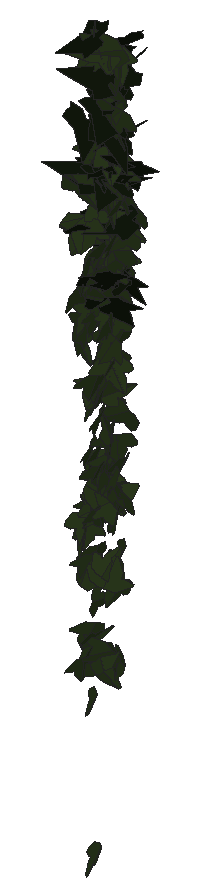
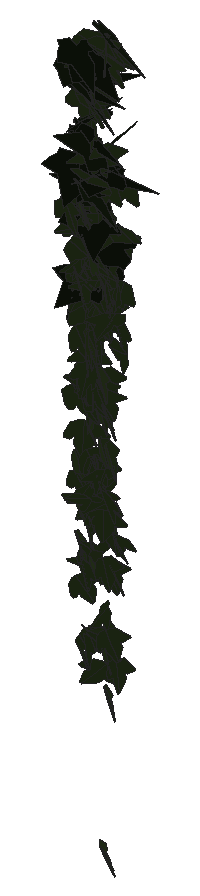
# SketchUp Ruby script. Lengths in inches.
U = 1.inch
M = Sketchup.active_model
def pt(a) = Geom::Point3d.new(a.map { |v| v * U })
def face(e, loops, mat)
  f = e.add_face(loops[0].map { |a| pt(a) })
  loops[1..].each { |l| e.add_face(l.map { |a| pt(a) }).erase! }
  f.material = f.back_material = mat if mat
  f
end
# faces: each face lists its corners as indices into pts; further lists are holes
def faces(e, pts, list, mat = nil) = list.each { |f| face(e, (f[0].is_a?(Array) ? f : [f]).map { |l| l.map { |i| pts[i] } }, mat) }
# xy, xz, yz: faces in a plane at the given z, y or x. An outline is a flat list of corners, or four numbers for a rectangle; further outlines are holes
def ring(l) = l.size == 4 ? [[l[0], l[1]], [l[2], l[1]], [l[2], l[3]], [l[0], l[3]]] : l.each_slice(2).to_a
def flat(e, list, mat, &to3) = list.each { |f| face(e, (f[0].is_a?(Array) ? f : [f]).map { |l| ring(l).map { |u, v| to3.(u, v) } }, mat) }
def xy(e, z, list, mat = nil) = flat(e, list, mat) { |x, y| [x, y, z] }
def xz(e, y, list, mat = nil) = flat(e, list, mat) { |x, z| [x, y, z] }
def yz(e, x, list, mat = nil) = flat(e, list, mat) { |y, z| [x, y, z] }
def lines(e, pts, list) = list.each { |a, b| e.add_line(pt(pts[a]), pt(pts[b])) }
# prism: a flat outline (further loops are holes) pulled along v
def prism(e, loops, v, mat = nil)
  f = face(e, loops, mat); d = Geom::Vector3d.new(v.map { |x| x * U })
  f.pushpull(f.normal.samedirection?(d) ? d.length : -d.length)
end
def box(e, o, s, mat = nil) = prism(e, [[o, [o[0] + s[0], o[1], o[2]], [o[0] + s[0], o[1] + s[1], o[2]], [o[0], o[1] + s[1], o[2]]]], [0, 0, s[2]], mat)
def at(x, y, z, deg = 0) = Geom::Transformation.translation(pt([x, y, z])) * Geom::Transformation.rotation(ORIGIN, Z_AXIS, deg.degrees)
def axes(o, x, y, z) = Geom::Transformation.new([*x, 0, *y, 0, *z, 0, *pt(o).to_a, 1])
def part(name) = M.definitions.add(name)
# library, detail: a bought-in or finely detailed component or shape, given as its bounding box
def library(name, o, s) = part(name).tap { |d| box(d.entities, o, s) }
def detail(e, o, s) = box(e.add_group.entities, o, s)
def put(e, d, t, mat = nil) = e.add_instance(d, t).tap { |i| i.material = mat if mat }
def group(e, t, mat = nil) = e.add_group.tap { |g| g.transformation = t; g.material = mat if mat }.entities
root = M.entities
M.materials.add("1026 AP 7946 SUNNY SIDE UP").color = [254, 231, 186]
M.materials.add("efeu1").color = [18, 25, 13]
M.materials.add("efeu2").color = [43, 57, 29]
c1 = part("ivyleaf_10")
p = [[0,0.5,-0.03],[-0.0625,2.02,-0.43],[-0.19,2.01,-0.46],[-0.54,1.05,-0.29],[-0.52,0.625,-0.18],[-0.83,0.76,-0.28],
  [-1.16,0.64,-0.33],[-1.15,0.33,-0.24],[-0.77,-0.39,0.02],[-0.3,-0.51,0.16],[0.04,-0.48,0.23],[-0.02,2.01,-0.4375],
  [-0.06,2.01,-0.43],[0.04,-0.49,0.23],[0.67,-0.49,0.14],[1.38,0.36,-0.2],[1.375,0.51,-0.24],[0.81,0.65,-0.19],
  [0.62,0.59,-0.15],[0.6,1.09,-0.28],[0.5,1.23,-0.31]]
faces(c1.entities,p,[[0,1,2,3,4,5,6,7,8,9,10],[11,12,0,13,14,15,16,17,18,19,20]],"efeu2")
c2 = part("ivyleaf_9")
p = [[1.54,2.16,1.25],[1.36,2.04,1.19],[-0.21,0.99,0.68],[-0.71,1.11,0.82],[-0.85,0.86,0.67],[-0.8,0.17,0.21],
  [-0.9,-0.01,0.1],[-0.67,-0.16,-0.02],[-0.08,-0.08,-0.05],[-0.03,-0.6,-0.4],[0.65,-0.88,-0.66],[0.83,-0.6,-0.49],
  [1.29,-0.42,-0.43],[1.8125,-0.07,-0.26],[1.21,0.44,0.15]]
faces(c2.entities,p,[[0,1,2,3,4,5,6,7,8,9,10,11,12,13,14]],"efeu1")
put(root,c1,axes([98.29,212.76,264.19],[-0.22971,-0.152,0.11857],[-0.04918,-0.12497,-0.21008],[0.29657,-0.13846,0.057]),"1026 AP 7946 SUNNY SIDE UP")
put(root,c1,axes([98.25,213.08,261.87],[0.0644,-0.18084,-0.07279],[-0.03638,0.06251,-0.19678],[0.32455,0.04289,-0.00761]),"1026 AP 7946 SUNNY SIDE UP")
put(root,c1,axes([98.24,212.66,256.42],[-0.06854,-0.19891,-0.02661],[0.0175,0.02284,-0.20955],[0.31468,-0.04459,0.00586]),"1026 AP 7946 SUNNY SIDE UP")
put(root,c1,axes([98.11,212.79,258.72],[0.18384,-0.12088,0.13408],[0.13954,-0.09617,-0.17379],[0.24285,0.14677,-0.00164]),"1026 AP 7946 SUNNY SIDE UP")
put(root,c1,axes([98.26,212.58,262.52],[0.22707,-0.1538,-0.09871],[-0.05451,0.0957,-0.21347],[0.27893,0.14391,0.03864]),"1026 AP 7946 SUNNY SIDE UP")
put(root,c1,axes([98.16,212.81,258.85],[0.32191,-0.01328,0.03541],[0.0514,-0.02499,-0.21022],[0.02698,0.20609,-0.02198]),"1026 AP 7946 SUNNY SIDE UP")
put(root,c2,axes([98.14,212.84,266.04],[-0.01817,-0.22293,0.11408],[-0.01715,-0.11156,-0.23057],[0.39191,-0.01522,-0.0048]),"1026 AP 7946 SUNNY SIDE UP")
put(root,c2,axes([98.54,212.66,265.22],[-0.21843,0.05872,0.17567],[-0.27405,0.03415,-0.14884],[-0.10817,-0.2051,0.02234]),"1026 AP 7946 SUNNY SIDE UP")
put(root,c1,axes([98.09,212.75,262.18],[-0.13955,0.04564,-0.21141],[0.16862,-0.18208,-0.09045],[-0.28479,-0.13017,0.05004]),"1026 AP 7946 SUNNY SIDE UP")
put(root,c1,axes([98.29,212.8,258.22],[-0.09401,-0.19406,0.04191],[-0.00495,-0.0427,-0.20922],[0.3121,-0.05913,0.0093]),"1026 AP 7946 SUNNY SIDE UP")
put(root,c1,axes([98.3,212.81,256.99],[-0.12749,-0.17983,0.05348],[-0.01708,-0.05307,-0.20319],[0.29427,-0.08099,0.01138]),"1026 AP 7946 SUNNY SIDE UP")
put(root,c1,axes([98.24,212.52,263.16],[-0.01748,-0.19451,-0.168],[0.06344,0.15869,-0.19825],[0.39292,-0.03427,0.02454]),"1026 AP 7946 SUNNY SIDE UP")
put(root,c1,axes([98.29,212.92,258.35],[-0.0743,-0.19922,0.00153],[0.00432,-0.00334,-0.21091],[0.31325,-0.0472,0.00327]),"1026 AP 7946 SUNNY SIDE UP")
put(root,c1,axes([98.15,212.93,262.87],[0.15264,0.20177,0.06018],[0.05518,0.04659,-0.23011],[-0.32514,0.10263,-0.0108]),"1026 AP 7946 SUNNY SIDE UP")
put(root,c1,axes([98.27,212.92,259.6],[0.24617,-0.13627,-0.02644],[-0.02313,0.021,-0.2136],[0.21659,0.15712,0.00724]),"1026 AP 7946 SUNNY SIDE UP")
put(root,c1,axes([98.27,212.91,263.41],[0.16233,-0.20482,-0.05122],[0.00816,0.05655,-0.23401],[0.33088,0.09909,0.0309]),"1026 AP 7946 SUNNY SIDE UP")
put(root,c1,axes([98.29,212.88,261.1],[0.17184,-0.19541,-0.00772],[-0.00907,0.00409,-0.23061],[0.30729,0.1094,-0.00249]),"1026 AP 7946 SUNNY SIDE UP")
put(root,c1,axes([98.26,212.67,257.9],[0.28096,-0.11428,0.0199],[-0.00721,0.02968,0.21746],[-0.18228,-0.17733,0.02207]),"1026 AP 7946 SUNNY SIDE UP")
put(root,c1,axes([98.34,212.9,259.1875],[-0.23044,-0.1348,-0.00393],[0.02391,-0.01147,-0.20406],[0.2276,-0.13528,0.01745]),"1026 AP 7946 SUNNY SIDE UP")
put(root,c1,axes([98.21,212.58,265.1],[-0.30673,-0.00524,-0.11432],[0.17984,-0.03596,-0.19065],[-0.0235,-0.20674,0.03309]),"1026 AP 7946 SUNNY SIDE UP")
put(root,c1,axes([98.34,212.74,260.3],[0.08197,-0.21019,-0.01942],[-0.00422,0.01752,-0.22299],[0.33164,0.05218,0.00196]),"1026 AP 7946 SUNNY SIDE UP")
put(root,c1,axes([98.32,212.76,263.54],[-0.00491,0.19552,-0.13215],[-0.06305,-0.12793,-0.19892],[-0.36322,0.01956,0.03632]),"1026 AP 7946 SUNNY SIDE UP")
put(root,c1,axes([98.41,212.92,261.34],[-0.23131,-0.1322,0.10215],[-0.04616,-0.11069,-0.19607],[0.25644,-0.13918,0.05685]),"1026 AP 7946 SUNNY SIDE UP")
put(root,c1,axes([98.26,212.66,264.32],[0.37558,0.0164,0.01636],[0.02822,-0.0215,-0.23658],[-0.02517,0.22072,-0.02113]),"1026 AP 7946 SUNNY SIDE UP")
put(root,c1,axes([98.46,212.72,267.62],[-0.15758,0.12687,0.17889],[-0.19353,0.12074,-0.16592],[-0.29632,-0.14632,0.01323]),"1026 AP 7946 SUNNY SIDE UP")
put(root,c1,axes([98.32,212.85,257.47],[0.00636,-0.06188,-0.20073],[0.06148,0.19116,-0.0607],[0.31498,-0.03607,0.0159]),"1026 AP 7946 SUNNY SIDE UP")
put(root,c2,axes([98.57,212.6,267.8],[-0.29349,0.1754,-0.0108],[-0.00675,-0.02125,-0.26328],[-0.29842,-0.17203,0.01658]),"1026 AP 7946 SUNNY SIDE UP")
put(root,c1,axes([98.4,212.84,265.7],[-0.1176,-0.21924,0.09],[0.01541,-0.09572,-0.23605],[0.37151,-0.06543,0.03828]),"1026 AP 7946 SUNNY SIDE UP")
put(root,c1,axes([98.44,212.81,267.4],[0.32445,-0.06472,-0.08538],[-0.13908,0.00256,-0.21468],[0.10328,0.20676,-0.02089]),"1026 AP 7946 SUNNY SIDE UP")
put(root,c1,axes([98.32,212.92,260],[0.10546,0.20612,0.01823],[0.00051,0.01727,-0.22314],[-0.32515,0.06688,0.00557]),"1026 AP 7946 SUNNY SIDE UP")
put(root,c1,axes([98.4,212.76,256.75],[0.06758,-0.19814,-0.01738],[-0.00061,0.01602,-0.20875],[0.31254,0.04287,0.00335]),"1026 AP 7946 SUNNY SIDE UP")
put(root,c2,axes([98.12,212.7,264.03],[0.2292,0.15255,-0.11025],[0.09916,0.08819,0.21888],[0.2983,-0.14653,0.01196]),"1026 AP 7946 SUNNY SIDE UP")
put(root,c1,axes([98.42,212.92,261.49],[-0.0993,-0.20231,0.06325],[0.01792,-0.06842,-0.21653],[0.33248,-0.05673,0.03056]),"1026 AP 7946 SUNNY SIDE UP")
put(root,c1,axes([98.48,212.74,262.78],[-0.16529,-0.15216,0.13866],[-0.05787,-0.13573,-0.18729],[0.31505,-0.10476,0.03834]),"1026 AP 7946 SUNNY SIDE UP")
put(root,c1,axes([98.62,212.72,267.54],[0.20334,-0.01781,-0.20681],[-0.32888,-0.01482,-0.12751],[-0.00553,0.22662,-0.0214]),"1026 AP 7946 SUNNY SIDE UP")
put(root,c1,axes([98.45,212.84,259.18],[0.02115,0.12114,-0.15666],[-0.11695,-0.13542,-0.12685],[-0.30275,0.06077,0.03806]),"1026 AP 7946 SUNNY SIDE UP")
put(root,c2,axes([98.55,213.04,267.42],[-0.01764,0.14972,-0.1576],[-0.0575,-0.1486,-0.15923],[-0.35413,0.01667,0.0337]),"1026 AP 7946 SUNNY SIDE UP")
put(root,c1,axes([98.45,212.94,263.88],[0.0211,-0.2373,0.00856],[-0.01113,-0.01007,-0.24479],[0.37327,0.01311,-0.00778]),"1026 AP 7946 SUNNY SIDE UP")
put(root,c1,axes([98.45,212.65,255.84],[0.12871,-0.1796,-0.04971],[-0.03129,0.04283,-0.20308],[0.29033,0.08424,0.00015]),"1026 AP 7946 SUNNY SIDE UP")
put(root,c1,axes([98.47,212.68,261.59],[-0.08202,-0.216,0.00735],[-0.00232,-0.00825,-0.22897],[0.33989,-0.05218,0.00021]),"1026 AP 7946 SUNNY SIDE UP")
put(root,c1,axes([98.43,212.75,253.03],[0.18468,-0.17561,0.0376],[0.01679,-0.03789,-0.21751],[0.28185,0.11732,-0.01168]),"1026 AP 7946 SUNNY SIDE UP")
put(root,c1,axes([98.48,212.95,263.35],[-0.11362,-0.21292,0.0654],[0.00117,-0.06825,-0.23095],[0.34991,-0.06891,0.02201]),"1026 AP 7946 SUNNY SIDE UP")
put(root,c2,axes([98.67,212.83,266.93],[-0.13402,-0.01059,0.22062],[-0.3224,-0.08292,-0.08356],[0.13757,-0.20465,0.01911]),"1026 AP 7946 SUNNY SIDE UP")
put(root,c1,axes([98.49,212.76,262.75],[-0.00318,-0.22617,0.04436],[0.0058,-0.04437,-0.23323],[0.36235,-0.00127,0.00412]),"1026 AP 7946 SUNNY SIDE UP")
put(root,c1,axes([98.39,212.63,256.82],[0.03832,-0.12765,0.1596],[0.03869,0.1575,0.13002],[-0.31415,0.00383,0.03548]),"1026 AP 7946 SUNNY SIDE UP")
put(root,c1,axes([98.5,212.7,260.34],[0.06741,-0.21819,-0.02668],[-0.00984,0.0239,-0.22893],[0.34512,0.0433,-0.00131]),"1026 AP 7946 SUNNY SIDE UP")
put(root,c1,axes([98.5,212.8,259.97],[-0.2697,0.13388,-0.00878],[-0.00333,-0.01777,-0.2237],[-0.21099,-0.17085,0.01476]),"1026 AP 7946 SUNNY SIDE UP")
put(root,c2,axes([98.41,212.76,265.45],[0.31349,0.13977,0.00154],[0.02054,-0.01661,-0.2472],[-0.23637,0.18392,-0.01943]),"1026 AP 7946 SUNNY SIDE UP")
put(root,c2,axes([98.68,212.85,265.05],[-0.1762,0.19802,-0.02045],[-0.00038,-0.02457,-0.23938],[-0.33816,-0.10315,0.01093]),"1026 AP 7946 SUNNY SIDE UP")
put(root,c1,axes([98.46,212.87,264.55],[0.20199,0.18711,-0.02128],[-0.01911,-0.01929,-0.23766],[-0.31931,0.11952,0.00076]),"1026 AP 7946 SUNNY SIDE UP")
put(root,c1,axes([98.43,212.98,263.4],[0.20222,0.17425,0.02367],[0.03433,0.01017,-0.22553],[-0.29572,0.12034,-0.01]),"1026 AP 7946 SUNNY SIDE UP")
put(root,c1,axes([98.46,212.63,259.61],[0.00453,0.1569,0.18599],[0.00817,0.17957,-0.16061],[-0.37495,0.00581,-0.00125]),"1026 AP 7946 SUNNY SIDE UP")
put(root,c1,axes([98.53,212.88,258.31],[0.09902,-0.18601,0.06887],[0.01632,-0.06806,-0.20237],[0.31094,0.06281,-0.01131]),"1026 AP 7946 SUNNY SIDE UP")
put(root,c1,axes([98.31,212.69,263.01],[-0.16068,0.05872,0.20743],[0.31684,-0.05539,0.11527],[0.12993,0.20769,-0.02457]),"1026 AP 7946 SUNNY SIDE UP")
put(root,c1,axes([98.35,212.85,259.41],[0.16698,0.11056,0.17086],[0.15036,0.13582,-0.15615],[-0.27406,0.14188,0.01843]),"1026 AP 7946 SUNNY SIDE UP")
put(root,c1,axes([98.54,212.77,260.05],[0.07045,-0.20519,-0.05876],[0.00231,0.05739,-0.2156],[0.33437,0.04283,0.01387]),"1026 AP 7946 SUNNY SIDE UP")
put(root,c2,axes([98.74,212.79,266.62],[-0.13603,0.17689,0.13039],[-0.09173,0.10667,-0.20636],[-0.35056,-0.09655,0.0034]),"1026 AP 7946 SUNNY SIDE UP")
put(root,c1,axes([98.79,212.75,267.59],[-0.18146,-0.02474,0.21694],[-0.30435,-0.09875,-0.11536],[0.16684,-0.20704,0.02552]),"1026 AP 7946 SUNNY SIDE UP")
put(root,c1,axes([98.49,212.72,265.05],[-0.34821,0.02393,-0.05338],[0.08016,-0.02618,-0.22042],[-0.04978,-0.20954,0.01843]),"1026 AP 7946 SUNNY SIDE UP")
put(root,c1,axes([98.54,212.69,259.25],[-0.0547,-0.1988,-0.06869],[0.03334,0.06276,-0.20732],[0.32746,-0.0396,0.00963]),"1026 AP 7946 SUNNY SIDE UP")
put(root,c1,axes([98.55,213,262.38],[0.13716,-0.20864,-0.00904],[-0.00331,0.00734,-0.23292],[0.32826,0.08725,0.00143]),"1026 AP 7946 SUNNY SIDE UP")
put(root,c2,axes([98.56,212.88,264.54],[0.22407,0.15525,-0.0973],[-0.08442,-0.07945,-0.21887],[-0.29531,0.14051,-0.01126]),"1026 AP 7946 SUNNY SIDE UP")
put(root,c1,axes([98.8,212.78,266.64],[-0.14241,0.01609,-0.22262],[-0.31485,0.09723,0.08943],[0.16268,0.20226,-0.02179]),"1026 AP 7946 SUNNY SIDE UP")
put(root,c1,axes([98.75,212.6,256.8],[-0.21755,-0.02541,0.16831],[-0.24391,-0.05432,-0.14423],[0.09063,-0.2072,0.01586]),"1026 AP 7946 SUNNY SIDE UP")
put(root,c1,axes([98.54,212.91,263.25],[-0.05203,-0.19356,0.12847],[0.05525,-0.12983,-0.19703],[0.35877,-0.00808,0.04898]),"1026 AP 7946 SUNNY SIDE UP")
put(root,c1,axes([98.29,212.87,263.54],[-0.01317,-0.03736,-0.21087],[0.30872,-0.08315,0.00808],[-0.1413,-0.17819,0.03731]),"1026 AP 7946 SUNNY SIDE UP")
put(root,c1,axes([98.66,212.63,259.4],[0.25898,-0.03648,-0.11675],[-0.18808,-0.0011,-0.16628],[0.04935,0.18726,-0.02101]),"1026 AP 7946 SUNNY SIDE UP")
put(root,c1,axes([98.62,212.76,262.41],[0.19891,-0.13599,-0.13967],[-0.0746,0.13427,-0.18462],[0.2917,0.12707,0.04802]),"1026 AP 7946 SUNNY SIDE UP")
put(root,c2,axes([98.83,212.875,266.02],[-0.07929,-0.01751,-0.23],[-0.35915,-0.03705,0.05202],[-0.06788,0.21648,-0.00657]),"1026 AP 7946 SUNNY SIDE UP")
put(root,c1,axes([98.56,213,261.82],[-0.16417,-0.18385,-0.07249],[0.06126,0.05757,-0.21741],[0.30281,-0.11132,0.00469]),"1026 AP 7946 SUNNY SIDE UP")
put(root,c1,axes([98.57,212.93,262.33],[0.0441,-0.22086,-0.0545],[0.0189,0.05341,-0.22828],[0.35615,0.02451,0.01886]),"1026 AP 7946 SUNNY SIDE UP")
put(root,c1,axes([98.56,212.96,263.54],[0.34388,-0.06462,-0.01762],[-0.03387,-0.01132,-0.22709],[0.10764,0.20286,-0.01515]),"1026 AP 7946 SUNNY SIDE UP")
put(root,c1,axes([98.59,212.65,261],[0.07606,-0.21281,-0.02731],[-0.00535,0.02518,-0.22466],[0.33693,0.04844,0.0026]),"1026 AP 7946 SUNNY SIDE UP")
put(root,c1,axes([98.625,212.93,263.56],[-0.29347,-0.13998,0.02087],[-0.00932,-0.02708,-0.23978],[0.22238,-0.18586,0.01749]),"1026 AP 7946 SUNNY SIDE UP")
put(root,c1,axes([98.59,212.69,259.99],[-0.14589,-0.19351,-0.03192],[0.02549,0.02536,-0.2209],[0.30683,-0.09412,0.00318]),"1026 AP 7946 SUNNY SIDE UP")
put(root,c1,axes([98.83,212.95,263.91],[-0.16824,0.02149,0.21702],[-0.33044,-0.03867,-0.10618],[0.03933,-0.23298,0.03623]),"1026 AP 7946 SUNNY SIDE UP")
put(root,c1,axes([98.48,212.77,256.35],[-0.23899,-0.05882,-0.10548],[0.1652,0.01912,-0.16209],[0.10107,-0.17033,0.01554]),"1026 AP 7946 SUNNY SIDE UP")
put(root,c2,axes([98.87,212.97,266.875],[-0.20248,0.08561,0.17261],[-0.24506,0.07146,-0.15504],[-0.18691,-0.18643,0.0163]),"1026 AP 7946 SUNNY SIDE UP")
put(root,c2,axes([98.73,212.68,264.93],[-0.13027,0.21192,-0.06355],[0.02841,-0.06,-0.24209],[-0.37381,-0.07841,0.00375]),"1026 AP 7946 SUNNY SIDE UP")
put(root,c2,axes([98.81,212.92,263.43],[-0.31796,0.10225,-0.00173],[-0.02754,-0.03576,-0.22508],[-0.17146,-0.18388,0.03936]),"1026 AP 7946 SUNNY SIDE UP")
put(root,c1,axes([98.62,212.71,261.46],[0.04827,-0.18386,-0.12807],[0.01233,0.12528,-0.18974],[0.34785,0.02107,0.0245]),"1026 AP 7946 SUNNY SIDE UP")
put(root,c1,axes([98.69,212.82,266.11],[-0.26979,0.14287,0.07169],[-0.10595,0.02751,-0.22737],[-0.24456,-0.16953,0.01941]),"1026 AP 7946 SUNNY SIDE UP")
put(root,c1,axes([98.63,212.94,259.07],[0.17358,-0.16747,-0.06473],[-0.02321,0.06394,-0.20504],[0.27977,0.10921,0.02315]),"1026 AP 7946 SUNNY SIDE UP")
put(root,c1,axes([98.52,212.91,259.47],[-0.0039,-0.03391,0.20392],[0.06767,0.18677,0.03863],[-0.32214,0.03965,0.00565]),"1026 AP 7946 SUNNY SIDE UP")
put(root,c1,axes([98.61,212.79,261.66],[0.18076,-0.18083,0.03539],[0.02664,-0.03186,-0.22509],[0.31166,0.1076,-0.00129]),"1026 AP 7946 SUNNY SIDE UP")
put(root,c2,axes([98.72,213.07,267.63],[-0.00026,0.20628,-0.07428],[0.00297,-0.07207,-0.22184],[-0.37092,-0.00072,-0.00172]),"1026 AP 7946 SUNNY SIDE UP")
put(root,c2,axes([98.53,212.83,265.76],[-0.02895,0.20921,-0.09732],[-0.01141,0.09339,0.22602],[0.38892,0.01831,-0.00062]),"1026 AP 7946 SUNNY SIDE UP")
put(root,c1,axes([98.81,212.96,264.77],[-0.12362,0.08842,0.1741],[-0.25298,0.07363,-0.11409],[-0.18347,-0.1611,0.04002]),"1026 AP 7946 SUNNY SIDE UP")
put(root,c1,axes([98.68,212.79,260.11],[-0.11545,-0.18541,0.08634],[0.00568,-0.09136,-0.20296],[0.32057,-0.06516,0.03469]),"1026 AP 7946 SUNNY SIDE UP")
put(root,c1,axes([98.68,213.04,259.4375],[0.19254,0.14351,0.03527],[-0.0485,-0.01695,0.19519],[0.2445,-0.11638,0.01094]),"1026 AP 7946 SUNNY SIDE UP")
put(root,c1,axes([98.7,212.81,259.66],[0.27995,-0.07665,-0.08339],[-0.0837,0.07467,-0.19407],[0.15345,0.18057,0.04628]),"1026 AP 7946 SUNNY SIDE UP")
put(root,c1,axes([98.78,212.49,256.61],[0.20979,0.01129,0.17228],[-0.22548,0.12189,0.10184],[-0.15497,-0.16207,0.08504]),"1026 AP 7946 SUNNY SIDE UP")
put(root,c1,axes([98.68,212.89,264.12],[0.1125,-0.22648,0.01529],[0.00214,-0.01648,-0.24475],[0.35701,0.07147,-0.00335]),"1026 AP 7946 SUNNY SIDE UP")
put(root,c2,axes([98.63,212.92,265.22],[-0.15691,-0.20919,0.08344],[-0.00227,-0.08932,-0.23655],[0.35339,-0.09345,0.03553]),"1026 AP 7946 SUNNY SIDE UP")
put(root,c1,axes([98.75,212.84,267.19],[0.21967,-0.18607,-0.14023],[-0.08683,0.12626,-0.2373],[0.35095,0.14771,0.02906]),"1026 AP 7946 SUNNY SIDE UP")
put(root,c1,axes([98.71,212.71,260.65],[-0.10821,0.19681,0.01786],[0.01391,-0.01219,0.22126],[0.33466,0.06415,-0.00342]),"1026 AP 7946 SUNNY SIDE UP")
put(root,c2,axes([98.61,212.82,266.36],[-0.11875,-0.19783,0.13988],[0.01707,-0.14615,-0.21225],[0.37791,-0.05556,0.05354]),"1026 AP 7946 SUNNY SIDE UP")
put(root,c1,axes([98.63,212.83,265.61],[0.17086,0.19212,-0.02318],[-0.00369,-0.0261,-0.2323],[-0.32867,0.10016,-0.00944]),"1026 AP 7946 SUNNY SIDE UP")
put(root,c1,axes([98.78,212.79,266.63],[0.23094,-0.15536,-0.1016],[-0.12471,0.05879,-0.21967],[0.28082,0.15387,-0.014]),"1026 AP 7946 SUNNY SIDE UP")
put(root,c1,axes([98.73,212.96,261.65],[0.03055,-0.22032,-0.0356],[-0.0079,0.03299,-0.22765],[0.35027,0.01996,-0.00203]),"1026 AP 7946 SUNNY SIDE UP")
put(root,c2,axes([98.64,212.47,263.5625],[0.22787,0.16303,0.03021],[0.04484,0.01198,-0.22551],[-0.27666,0.13622,-0.01167]),"1026 AP 7946 SUNNY SIDE UP")
put(root,c1,axes([98.56,212.96,265.25],[0.34479,0.06424,0.07957],[0.11629,0.02098,-0.23527],[-0.10626,0.23141,0.00071]),"1026 AP 7946 SUNNY SIDE UP")
put(root,c1,axes([98.67,212.8,264.37],[0.37011,0.06859,-0.0088],[0.00183,0.02775,0.25127],[0.10875,-0.23391,0.02572]),"1026 AP 7946 SUNNY SIDE UP")
put(root,c1,axes([98.75,212.84,262.74],[-0.22899,-0.15956,0.08321],[0.01391,-0.11151,-0.20882],[0.28152,-0.12428,0.07801]),"1026 AP 7946 SUNNY SIDE UP")
put(root,c1,axes([98.75,212.98,262.4],[-0.06608,-0.21769,0.05134],[-0.00053,-0.0519,-0.22851],[0.35159,-0.04099,0.0093]),"1026 AP 7946 SUNNY SIDE UP")
put(root,c1,axes([98.73,212.91,264.71],[0.12622,-0.22115,0.06583],[0.0117,-0.06647,-0.24226],[0.36233,0.07918,-0.01511]),"1026 AP 7946 SUNNY SIDE UP")
put(root,c1,axes([98.7,212.93,258.22],[0.24763,-0.134,-0.01358],[0.01432,0.02969,-0.21082],[0.21112,0.15516,0.03023]),"1026 AP 7946 SUNNY SIDE UP")
put(root,c1,axes([98.68,212.77,264.86],[-0.04794,0.20085,-0.04463],[0.00065,-0.04467,-0.21768],[-0.34914,-0.02766,0.00572]),"1026 AP 7946 SUNNY SIDE UP")
put(root,c1,axes([98.78,212.93,257.88],[-0.10308,-0.16725,0.09671],[-0.01814,-0.09659,-0.18427],[0.30177,-0.06294,0.02196]),"1026 AP 7946 SUNNY SIDE UP")
put(root,c2,axes([98.51,212.73,265.1],[0.12238,0.03821,0.20927],[0.30645,0.07404,-0.08596],[-0.14088,0.19425,-0.00519]),"1026 AP 7946 SUNNY SIDE UP")
put(root,c1,axes([98.72,212.66,263.63],[-0.13153,-0.20394,-0.09686],[0.07172,0.08155,-0.22635],[0.34497,-0.09471,0.01013]),"1026 AP 7946 SUNNY SIDE UP")
put(root,c1,axes([98.77,212.75,262],[0.03354,-0.15201,-0.11535],[-0.02207,0.10496,-0.16265],[0.31359,0.02365,0.00089]),"1026 AP 7946 SUNNY SIDE UP")
put(root,c1,axes([98.7,212.65,259.98],[0.03428,-0.18912,-0.11405],[0.07805,0.11158,-0.18747],[0.33475,-0.00665,0.05539]),"1026 AP 7946 SUNNY SIDE UP")
put(root,c1,axes([98.81,212.71,266.5],[-0.3906,0.04949,0.02491],[-0.05289,-0.03922,-0.24794],[-0.07573,-0.22786,0.04466]),"1026 AP 7946 SUNNY SIDE UP")
put(root,c1,axes([98.69,212.9375,263.7],[0.0209,0.23419,0.01638],[-0.00322,0.01471,-0.24155],[-0.36894,0.01314,0.00304]),"1026 AP 7946 SUNNY SIDE UP")
put(root,c1,axes([98.77,212.99,263.51],[0.10375,-0.22146,-0.03169],[-0.01022,0.02884,-0.23788],[0.35115,0.06627,0.00244]),"1026 AP 7946 SUNNY SIDE UP")
put(root,c1,axes([98.68,212.97,263.71],[0.10517,0.22484,-0.00411],[0.01129,-0.00762,-0.24152],[-0.35345,0.06666,-0.00894]),"1026 AP 7946 SUNNY SIDE UP")
put(root,c1,axes([98.75,212.65,262.7],[0.01053,-0.20323,-0.11122],[0.04067,0.10684,-0.20713],[0.3587,-0.00615,0.02675]),"1026 AP 7946 SUNNY SIDE UP")
put(root,c2,axes([98.625,212.95,263.4],[0.35125,0.0455,-0.0102],[-0.00935,-0.02185,-0.22609],[-0.07858,0.20601,-0.01868]),"1026 AP 7946 SUNNY SIDE UP")
put(root,c1,axes([98.78,212.93,259.31],[0.10465,-0.19868,0.02779],[0.00269,-0.02904,-0.21589],[0.31551,0.06615,-0.00738]),"1026 AP 7946 SUNNY SIDE UP")
put(root,c1,axes([98.73,212.81,263.22],[-0.10536,-0.16948,-0.15713],[0.10925,0.13519,-0.18658],[0.34041,-0.09584,0.01124]),"1026 AP 7946 SUNNY SIDE UP")
put(root,c1,axes([98.92,212.85,264.27],[-0.27934,-0.03736,0.10375],[-0.14408,-0.05782,-0.17807],[0.10296,-0.18227,0.03232]),"1026 AP 7946 SUNNY SIDE UP")
put(root,c1,axes([98.8,212.73,256.7],[0.17778,-0.13533,-0.10292],[-0.02976,0.1085,-0.17418],[0.2621,0.10411,0.05004]),"1026 AP 7946 SUNNY SIDE UP")
put(root,c1,axes([98.82,212.62,262.39],[0.30686,-0.10936,-0.05909],[-0.06862,0.03694,-0.2254],[0.19516,0.18494,0.01366]),"1026 AP 7946 SUNNY SIDE UP")
put(root,c1,axes([99.01,212.75,261.15],[-0.24079,0.03006,0.17869],[-0.27509,-0.00258,-0.15883],[-0.02823,-0.23124,0.02362]),"1026 AP 7946 SUNNY SIDE UP")
put(root,c1,axes([98.91,212.76,256.58],[0.03559,-0.07173,-0.19489],[-0.13879,0.16733,-0.07542],[0.28559,0.09026,-0.01237]),"1026 AP 7946 SUNNY SIDE UP")
put(root,c1,axes([98.67,212.82,260.68],[0.14217,-0.11708,0.16583],[0.16135,-0.12493,-0.15309],[0.26917,0.13672,0.00418]),"1026 AP 7946 SUNNY SIDE UP")
put(root,c1,axes([98.82,212.92,260.12],[0.01703,-0.21715,0.01878],[-0.00151,-0.01953,-0.22409],[0.34282,0.0107,-0.00192]),"1026 AP 7946 SUNNY SIDE UP")
put(root,c1,axes([98.72,212.58,258.26],[0.1268,0.11607,-0.16041],[0.11494,0.13582,0.14918],[0.30269,-0.1002,0.01055]),"1026 AP 7946 SUNNY SIDE UP")
put(root,c1,axes([98.74,212.91,267.4],[0.06073,0.21645,-0.03463],[-0.00536,-0.03512,-0.23534],[-0.37221,0.03582,-0.00226]),"1026 AP 7946 SUNNY SIDE UP")
put(root,c1,axes([98.8,212.69,260.02],[0.2216,-0.15978,0.00383],[-0.01105,-0.01262,-0.22063],[0.27118,0.13005,-0.01212]),"1026 AP 7946 SUNNY SIDE UP")
put(root,c2,axes([98.91,213.15,267.3],[-0.17315,0.1561,-0.11154],[0.08441,-0.09426,-0.20073],[-0.3092,-0.11315,0.00767]),"1026 AP 7946 SUNNY SIDE UP")
put(root,c1,axes([98.83,212.77,260.58],[-0.23086,-0.16976,-0.01819],[0.0364,0.00199,-0.23061],[0.26573,-0.14775,0.01578]),"1026 AP 7946 SUNNY SIDE UP")
put(root,c2,axes([99.03,212.83,264.57],[-0.34236,0.08629,0.00319],[-0.03937,-0.04965,-0.2281],[-0.14112,-0.19548,0.0559]),"1026 AP 7946 SUNNY SIDE UP")
put(root,c2,axes([98.68,212.76,266.22],[0.03148,-0.24115,-0.06765],[-0.00538,0.06423,-0.2489],[0.39239,0.02023,0.00202]),"1026 AP 7946 SUNNY SIDE UP")
put(root,c1,axes([98.74,212.74,261.92],[-0.20703,-0.17092,-0.04716],[0.16049,-0.02074,-0.20473],[0.25192,-0.12725,0.09168]),"1026 AP 7946 SUNNY SIDE UP")
put(root,c1,axes([98.6,212.86,264.39],[0.12317,0.08607,0.2083],[0.2254,0.14078,-0.11842],[-0.27995,0.15122,-0.0037]),"1026 AP 7946 SUNNY SIDE UP")
put(root,c1,axes([98.93,212.75,259.62],[-0.27898,0.09001,0.08172],[-0.13354,0.00453,-0.20227],[-0.1325,-0.19409,0.0318]),"1026 AP 7946 SUNNY SIDE UP")
put(root,c1,axes([98.875,212.83,258.58],[0.10814,-0.18705,-0.06783],[-0.04151,0.0593,-0.20492],[0.30847,0.07355,-0.0038]),"1026 AP 7946 SUNNY SIDE UP")
put(root,c1,axes([98.74,212.67,261.37],[-0.0492,-0.08163,0.18534],[0.07168,0.16916,0.09475],[-0.31859,0.05066,-0.0073]),"1026 AP 7946 SUNNY SIDE UP")
put(root,c2,axes([98.8,212.92,265.41],[0.24725,0.1813,-0.02923],[-0.00817,-0.0343,-0.24671],[-0.28868,0.15625,-0.01805]),"1026 AP 7946 SUNNY SIDE UP")
put(root,c1,axes([98.99,213.04,264.65],[-0.24269,0.07124,0.11979],[-0.19143,0.01879,-0.16819],[-0.11603,-0.18,0.02692]),"1026 AP 7946 SUNNY SIDE UP")
put(root,c1,axes([98.75,212.59,258.07],[0.29932,0.07783,-0.06913],[0.08806,0.04416,0.20602],[0.14866,-0.18287,0.01717]),"1026 AP 7946 SUNNY SIDE UP")
put(root,c2,axes([98.74,212.56,263.11],[0.31879,0.12619,0.00813],[0.01913,-0.00612,-0.242],[-0.21359,0.18779,-0.00954]),"1026 AP 7946 SUNNY SIDE UP")
